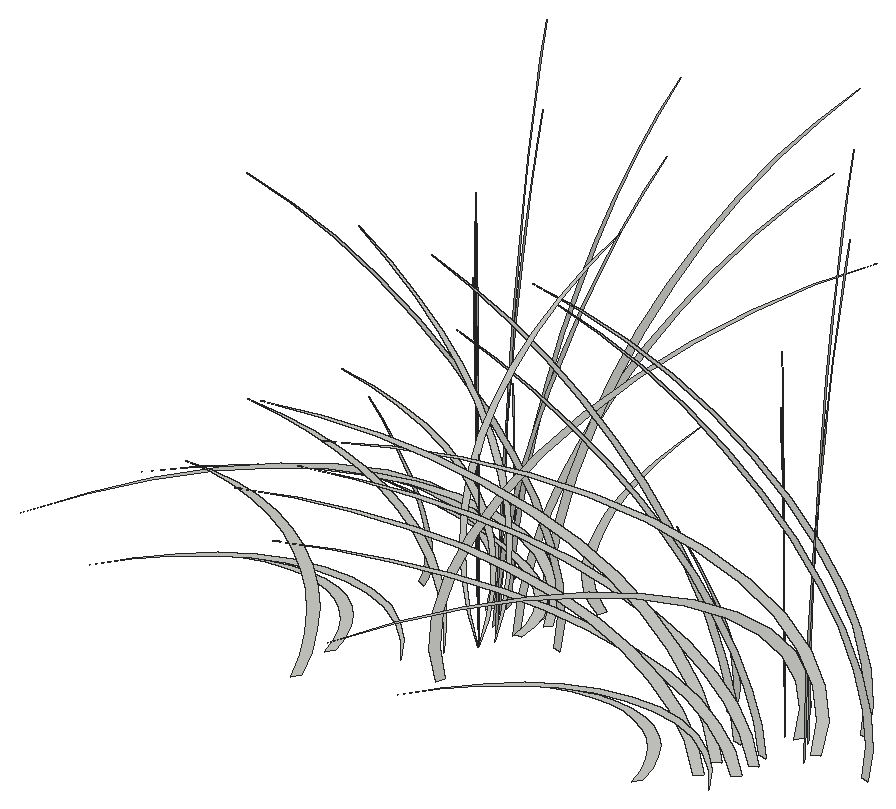
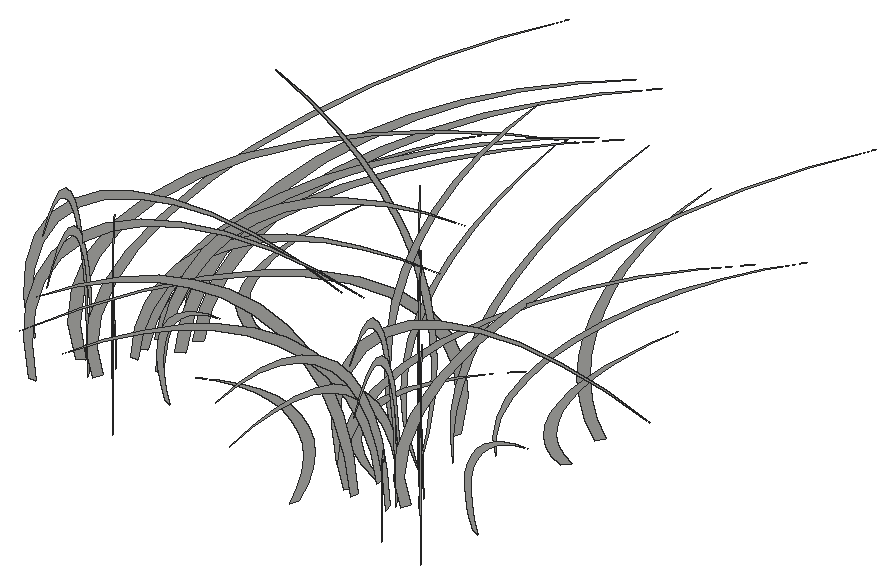
# SketchUp Ruby script. Lengths in inches.
U = 1.inch
M = Sketchup.active_model
def pt(a) = Geom::Point3d.new(a.map { |v| v * U })
def face(e, loops, mat)
  f = e.add_face(loops[0].map { |a| pt(a) })
  loops[1..].each { |l| e.add_face(l.map { |a| pt(a) }).erase! }
  f.material = f.back_material = mat if mat
  f
end
# faces: each face lists its corners as indices into pts; further lists are holes
def faces(e, pts, list, mat = nil) = list.each { |f| face(e, (f[0].is_a?(Array) ? f : [f]).map { |l| l.map { |i| pts[i] } }, mat) }
# xy, xz, yz: faces in a plane at the given z, y or x. An outline is a flat list of corners, or four numbers for a rectangle; further outlines are holes
def ring(l) = l.size == 4 ? [[l[0], l[1]], [l[2], l[1]], [l[2], l[3]], [l[0], l[3]]] : l.each_slice(2).to_a
def flat(e, list, mat, &to3) = list.each { |f| face(e, (f[0].is_a?(Array) ? f : [f]).map { |l| ring(l).map { |u, v| to3.(u, v) } }, mat) }
def xy(e, z, list, mat = nil) = flat(e, list, mat) { |x, y| [x, y, z] }
def xz(e, y, list, mat = nil) = flat(e, list, mat) { |x, z| [x, y, z] }
def yz(e, x, list, mat = nil) = flat(e, list, mat) { |y, z| [x, y, z] }
def lines(e, pts, list) = list.each { |a, b| e.add_line(pt(pts[a]), pt(pts[b])) }
# prism: a flat outline (further loops are holes) pulled along v
def prism(e, loops, v, mat = nil)
  f = face(e, loops, mat); d = Geom::Vector3d.new(v.map { |x| x * U })
  f.pushpull(f.normal.samedirection?(d) ? d.length : -d.length)
end
def box(e, o, s, mat = nil) = prism(e, [[o, [o[0] + s[0], o[1], o[2]], [o[0] + s[0], o[1] + s[1], o[2]], [o[0], o[1] + s[1], o[2]]]], [0, 0, s[2]], mat)
def at(x, y, z, deg = 0) = Geom::Transformation.translation(pt([x, y, z])) * Geom::Transformation.rotation(ORIGIN, Z_AXIS, deg.degrees)
def axes(o, x, y, z) = Geom::Transformation.new([*x, 0, *y, 0, *z, 0, *pt(o).to_a, 1])
def part(name) = M.definitions.add(name)
# library, detail: a bought-in or finely detailed component or shape, given as its bounding box
def library(name, o, s) = part(name).tap { |d| box(d.entities, o, s) }
def detail(e, o, s) = box(e.add_group.entities, o, s)
def put(e, d, t, mat = nil) = e.add_instance(d, t).tap { |i| i.material = mat if mat }
def group(e, t, mat = nil) = e.add_group.tap { |g| g.transformation = t; g.material = mat if mat }.entities
root = M.entities
g1 = group(root,at(461.7,262.6875,0))
p = [[-0.95,0.28,0],[-0.42,0.125,0],[0,0,2.01],[-0.17,0.05,4.04],[-0.93,0.27,6.02],[-2.27,0.66,7.92],
  [-4.14,1.21,9.68],[-6.5,1.9,11.26],[-9.3,2.72,12.62],[-12.46,3.64,13.73],[-15.91,4.65,14.5625],[-19.55,5.72,15.09],
  [-23.3125,6.82,15.31],[-27.08,7.92,15.2],[-23.38,6.84,15.22],[-19.72,5.77,14.94],[-16.17,4.73,14.37],[-12.83,3.75,13.51],
  [-9.77,2.86,12.39],[-7.0625,2.07,11.04],[-4.77,1.39,9.48],[-2.94,0.86,7.75],[-1.62,0.47,5.9],[-0.84,0.25,3.96],
  [-0.61,0.18,1.98]]
faces(g1,p,[[0,1,2,3,4,5,6,7,8,9,10,11,12,13,14,15,16,17,18,19,20,21,22,23,24]])
g2 = group(root,at(452.43,263.44,0))
p = [[-6.53,2.99,7.88],[-5.33,2.44,7.38],[-4.26,1.95,6.83],[-3.3,1.51,6.24],[-2.48,1.14,5.62],[-1.81,0.83,4.96],
  [-1.28,0.58,4.27],[-0.9,0.41,3.57],[-0.68,0.31,2.86],[-0.61,0.28,2.13],[-0.71,0.32,1.41],[-0.96,0.4375,0.7],
  [-1.37,0.625,0],[-0.84,0.38,0],[-0.39,0.18,0.71],[-0.11,0.05,1.43],[0,0,2.17],[-0.07,0.03,2.9],
  [-0.32,0.15,3.63],[-0.74,0.34,4.34],[-1.33,0.61,5.03],[-2.08,0.95,5.69],[-2.99,1.37,6.3125],[-4.04,1.85,6.89],
  [-5.22,2.39,7.41]]
faces(g2,p,[[0,1,2,3,4,5,6,7,8,9,10,11,12,13,14,15,16,17,18,19,20,21,22,23,24]])
g3 = group(root,at(455.19,263.66,0))
p = [[-10.66,12.98,9.9],[-9.23,11.23,9.83],[-7.82,9.52,9.59],[-6.46,7.86,9.18],[-5.18,6.3,8.61],[-3.99,4.86,7.88],
  [-2.93,3.57,7.02],[-2.02,2.46,6.03],[-1.27,1.54,4.95],[-0.6875,0.84,3.78],[-0.29,0.36,2.55],[-0.1,0.12,1.28],
  [-0.09,0.12,0],[0,0,1.3],[-0.125,0.15,2.61],[-0.47,0.57,3.875],[-1.02,1.24,5.09],[-1.77,2.15,6.21],
  [-2.69,3.28,7.22],[-3.78,4.6,8.1],[-5,6.09,8.82],[-6.33,7.71,9.37],[-7.74,9.43,9.74],[-9.2,11.19,9.92]]
faces(g3,p,[[0,1,2,3,4,5,6,7,8,9,10,11,12,13,14,15,16,17,18,19,20,21,22,23]])
g4 = group(root,at(456.45,263.9375,0))
p = [[-11.32,17.43,20.75],[-13.02,20.05,21.3],[-11.37,17.51,20.63],[-9.77,15.05,19.72],[-8.25,12.7,18.55],[-6.82,10.5,17.16],
  [-5.5,8.46,15.55],[-4.29,6.61,13.74],[-3.23,4.97,11.76],[-2.3125,3.56,9.62],[-1.55,2.39,7.35],[-0.96,1.47,4.97],
  [-0.54,0.83,2.51],[-0.29,0.45,0],[0,0,0],[-0.2,0.31,2.57],[-0.59,0.91,5.09],[-1.18,1.8125,7.53],
  [-1.94,2.99,9.85],[-2.88,4.43,12.03],[-3.98,6.12,14.04],[-5.22,8.04,15.86],[-6.59,10.15,17.46],[-8.08,12.44,18.82],
  [-9.66,14.88,19.92]]
faces(g4,p,[[0,1,2,3,4,5,6,7,8,9,10,11,12,13,14,15,16,17,18,19,20,21,22,23,24]])
g5 = group(root,at(452.33,267.16,0))
p = [[-4.56,5.55,16.02],[-3.72,4.53,15.01],[-2.97,3.62,13.89],[-2.31,2.81,12.69],[-1.73,2.11,11.42],[-1.26,1.54,10.08],
  [-0.89,1.09,8.6875],[-0.63,0.76,7.26],[-0.47,0.58,5.8],[-0.43,0.52,4.34],[-0.49,0.6,2.87],[-0.67,0.81,1.42],
  [-0.95,1.16,0],[-0.59,0.71,0],[-0.27,0.33,1.44],[-0.07,0.09,2.92],[0,0,4.41],[-0.05,0.0625,5.9],
  [-0.22,0.27,7.38],[-0.52,0.63,8.83],[-0.93,1.13,10.23],[-1.45,1.77,11.57],[-2.09,2.54,12.83],[-2.82,3.43,14.01],
  [-3.65,4.44,15.07]]
faces(g5,p,[[0,1,2,3,4,5,6,7,8,9,10,11,12,13,14,15,16,17,18,19,20,21,22,23,24]])
g6 = group(root,at(452.33,267.16,0))
p = [[-4.56,5.55,16.02],[-3.72,4.53,15.01],[-2.97,3.62,13.89],[-2.31,2.81,12.69],[-1.73,2.11,11.42],[-1.26,1.54,10.08],
  [-0.89,1.09,8.6875],[-0.63,0.76,7.26],[-0.47,0.58,5.8],[-0.43,0.52,4.34],[-0.49,0.6,2.87],[-0.67,0.81,1.42],
  [-0.95,1.16,0],[-0.59,0.71,0],[-0.27,0.33,1.44],[-0.07,0.09,2.92],[0,0,4.41],[-0.05,0.0625,5.9],
  [-0.22,0.27,7.38],[-0.52,0.63,8.83],[-0.93,1.13,10.23],[-1.45,1.77,11.57],[-2.09,2.54,12.83],[-2.82,3.43,14.01],
  [-3.65,4.44,15.07]]
faces(g6,p,[[0,1,2,3,4,5,6,7,8,9,10,11,12,13,14,15,16,17,18,19,20,21,22,23,24]])
g7 = group(root,at(456.02,264.74,0))
p = [[-0.37,-0.92,0],[-0.16,-0.41,0],[0,0,1.75],[-0.07,-0.17,3.51],[-0.36,-0.9,5.24],[-0.88,-2.19,6.89],
  [-1.61,-4,8.42],[-2.53,-6.28,9.8],[-3.61,-8.99,10.98],[-4.84,-12.04,11.95],[-6.18,-15.375,12.67],[-7.6,-18.9,13.13],
  [-9.06,-22.53,13.32],[-10.53,-26.18,13.23],[-9.09,-22.6,13.25],[-7.66,-19.06,13],[-6.29,-15.63,12.5],[-4.99,-12.41,11.75],
  [-3.8,-9.45,10.78],[-2.75,-6.83,9.6],[-1.85,-4.61,8.25],[-1.14,-2.84,6.75],[-0.63,-1.57,5.13],[-0.33,-0.8125,3.44],
  [-0.24,-0.59,1.72]]
faces(g7,p,[[0,1,2,3,4,5,6,7,8,9,10,11,12,13,14,15,16,17,18,19,20,21,22,23,24]])
g8 = group(root,at(452.77,256.56,0))
p = [[-3.94,-6,6.7],[-3.22,-4.9,6.27],[-2.57,-3.91,5.81],[-2,-3.04,5.31],[-1.5,-2.28,4.77],[-1.09,-1.66,4.21],
  [-0.77,-1.17,3.63],[-0.54,-0.83,3.03],[-0.41,-0.62,2.43],[-0.37,-0.5625,1.8125],[-0.43,-0.65,1.2],[-0.58,-0.88,0.59],
  [-0.83,-1.26,0],[-0.51,-0.77,0],[-0.23,-0.36,0.6],[-0.0625,-0.1,1.22],[0,0,1.84],[-0.04,-0.07,2.47],
  [-0.19,-0.29,3.09],[-0.45,-0.68,3.69],[-0.8,-1.22,4.28],[-1.26,-1.91,4.84],[-1.81,-2.75,5.37],[-2.44,-3.71,5.86],
  [-3.16,-4.8,6.3]]
faces(g8,p,[[0,1,2,3,4,5,6,7,8,9,10,11,12,13,14,15,16,17,18,19,20,21,22,23,24]])
g9 = group(root,at(455.54,257.25,0))
p = [[-9.23,-14.04,8.41],[-7.99,-12.15,8.36],[-6.77,-10.29,8.15],[-5.59,-8.5,7.8],[-4.48,-6.8125,7.32],[-3.46,-5.26,6.7],
  [-2.54,-3.86,5.97],[-1.75,-2.66,5.13],[-1.09,-1.67,4.2],[-0.59,-0.9,3.21],[-0.25,-0.39,2.16],[-0.08,-0.125,1.09],
  [-0.08,-0.125,0],[0,0,1.11],[-0.11,-0.16,2.21],[-0.4,-0.61,3.29],[-0.88,-1.34,4.32],[-1.53,-2.33,5.28],
  [-2.33,-3.55,6.14],[-3.27,-4.98,6.88],[-4.33,-6.59,7.5],[-5.48,-8.34,7.97],[-6.7,-10.19,8.28],[-7.96,-12.11,8.43]]
faces(g9,p,[[0,1,2,3,4,5,6,7,8,9,10,11,12,13,14,15,16,17,18,19,20,21,22,23]])
g10 = group(root,at(457.5,262.32,0))
p = [[-11.32,17.43,16.73],[-13.02,20.05,17.17],[-11.37,17.51,16.64],[-9.77,15.05,15.9],[-8.25,12.7,14.96],[-6.82,10.5,13.84],
  [-5.5,8.46,12.54],[-4.29,6.61,11.08],[-3.23,4.97,9.48],[-2.3125,3.56,7.76],[-1.55,2.39,5.92],[-0.96,1.47,4.01],
  [-0.54,0.83,2.02],[-0.29,0.45,0],[0,0,0],[-0.2,0.31,2.07],[-0.59,0.91,4.1],[-1.18,1.8125,6.07],
  [-1.94,2.99,7.94],[-2.88,4.43,9.7],[-3.98,6.12,11.33],[-5.22,8.04,12.79],[-6.59,10.15,14.08],[-8.08,12.44,15.17],
  [-9.66,14.88,16.0625]]
faces(g10,p,[[0,1,2,3,4,5,6,7,8,9,10,11,12,13,14,15,16,17,18,19,20,21,22,23,24]])
g11 = group(root,at(453.05,253.48,0))
p = [[-3.94,-6,13.62],[-3.22,-4.9,12.76],[-2.57,-3.91,11.81],[-2,-3.04,10.79],[-1.5,-2.28,9.7],[-1.09,-1.66,8.57],
  [-0.77,-1.17,7.38],[-0.54,-0.83,6.17],[-0.41,-0.62,4.93],[-0.37,-0.5625,3.6875],[-0.43,-0.65,2.44],[-0.58,-0.88,1.21],
  [-0.83,-1.26,0],[-0.51,-0.77,0],[-0.23,-0.36,1.22],[-0.0625,-0.1,2.48],[0,0,3.75],[-0.04,-0.07,5.02],
  [-0.19,-0.29,6.28],[-0.45,-0.68,7.51],[-0.8,-1.22,8.7],[-1.26,-1.91,9.84],[-1.81,-2.75,10.91],[-2.44,-3.71,11.9],
  [-3.16,-4.8,12.8125]]
faces(g11,p,[[0,1,2,3,4,5,6,7,8,9,10,11,12,13,14,15,16,17,18,19,20,21,22,23,24]])
g12 = group(root,at(459.52,264.9,0))
p = [[-0.5,-0.57,0],[-0.22,-0.25,0],[0,0,1.46],[-0.09,-0.1,2.93],[-0.49,-0.56,4.375],[-1.19,-1.35,5.75],
  [-2.17,-2.47,7.03],[-3.41,-3.89,8.18],[-4.88,-5.56,9.17],[-6.54,-7.45,9.98],[-8.36,-9.51,10.58],[-10.27,-11.69,10.97],
  [-12.24,-13.9375,11.125],[-14.23,-16.19,11.05],[-12.28,-13.98,11.0625],[-10.36,-11.79,10.86],[-8.5,-9.67,10.44],[-6.74,-7.67,9.82],
  [-5.13,-5.84,9.01],[-3.71,-4.22,8.02],[-2.51,-2.85,6.89],[-1.54,-1.76,5.64],[-0.85,-0.97,4.29],[-0.44,-0.5,2.88],
  [-0.32,-0.37,1.4375]]
faces(g12,p,[[0,1,2,3,4,5,6,7,8,9,10,11,12,13,14,15,16,17,18,19,20,21,22,23,24]])
g13 = group(root,at(459.52,264.9,0))
p = [[-0.5,-0.57,0],[-0.22,-0.25,0],[0,0,1.46],[-0.09,-0.1,2.93],[-0.49,-0.56,4.375],[-1.19,-1.35,5.75],
  [-2.17,-2.47,7.03],[-3.41,-3.89,8.18],[-4.88,-5.56,9.17],[-6.54,-7.45,9.98],[-8.36,-9.51,10.58],[-10.27,-11.69,10.97],
  [-12.24,-13.9375,11.125],[-14.23,-16.19,11.05],[-12.28,-13.98,11.0625],[-10.36,-11.79,10.86],[-8.5,-9.67,10.44],[-6.74,-7.67,9.82],
  [-5.13,-5.84,9.01],[-3.71,-4.22,8.02],[-2.51,-2.85,6.89],[-1.54,-1.76,5.64],[-0.85,-0.97,4.29],[-0.44,-0.5,2.88],
  [-0.32,-0.37,1.4375]]
faces(g13,p,[[0,1,2,3,4,5,6,7,8,9,10,11,12,13,14,15,16,17,18,19,20,21,22,23,24]])
g14 = group(root,at(456.41,264.57,0))
p = [[-6.07,19.87,18.05],[-6.99,22.87,18.53],[-6.1,19.96,17.95],[-5.25,17.16,17.15],[-4.43,14.49,16.14],[-3.66,11.97,14.93],
  [-2.95,9.65,13.53],[-2.31,7.54,11.96],[-1.73,5.67,10.23],[-1.24,4.06,8.37],[-0.83,2.72,6.39],[-0.51,1.68,4.32],
  [-0.29,0.94,2.18],[-0.16,0.52,0],[0,0,0],[-0.11,0.35,2.23],[-0.32,1.04,4.43],[-0.63,2.07,6.55],
  [-1.04,3.41,8.57],[-1.55,5.05,10.47],[-2.13,6.98,12.22],[-2.8,9.16,13.8],[-3.54,11.58,15.1875],[-4.34,14.1875,16.37],
  [-5.1875,16.96,17.33]]
faces(g14,p,[[0,1,2,3,4,5,6,7,8,9,10,11,12,13,14,15,16,17,18,19,20,21,22,23,24]])
g15 = group(root,at(455.35,266.52,0))
p = [[-4.56,5.55,7.88],[-3.72,4.53,7.38],[-2.97,3.62,6.83],[-2.31,2.81,6.24],[-1.73,2.11,5.62],[-1.26,1.54,4.96],
  [-0.89,1.09,4.27],[-0.63,0.76,3.57],[-0.47,0.58,2.86],[-0.43,0.52,2.13],[-0.49,0.6,1.41],[-0.67,0.81,0.7],
  [-0.95,1.16,0],[-0.59,0.71,0],[-0.27,0.33,0.71],[-0.07,0.09,1.43],[0,0,2.17],[-0.05,0.0625,2.9],
  [-0.22,0.27,3.63],[-0.52,0.63,4.34],[-0.93,1.13,5.03],[-1.45,1.77,5.69],[-2.09,2.54,6.3125],[-2.82,3.43,6.89],
  [-3.65,4.44,7.41]]
faces(g15,p,[[0,1,2,3,4,5,6,7,8,9,10,11,12,13,14,15,16,17,18,19,20,21,22,23,24]])
g16 = group(root,at(456.64,261.91,0))
p = [[-6.74,8.21,19.61],[-5.67,6.9,18.16],[-4.68,5.7,16.67],[-3.78,4.6,15.125],[-2.98,3.62,13.55],[-2.27,2.76,11.93],
  [-1.65,2.01,10.28],[-1.14,1.39,8.61],[-0.72,0.88,6.91],[-0.41,0.5,5.2],[-0.2,0.24,3.47],[-0.09,0.11,1.74],
  [-0.09,0.11,0],[0,0,1.74],[-0.03,0.04,3.49],[-0.1875,0.23,5.23],[-0.46,0.56,6.96],[-0.85,1.04,8.67],
  [-1.36,1.66,10.36],[-1.98,2.42,12.01],[-2.72,3.3125,13.63],[-3.57,4.35,15.21],[-4.52,5.51,16.73],[-5.58,6.8,18.2]]
faces(g16,p,[[0,1,2,3,4,5,6,7,8,9,10,11,12,13,14,15,16,17,18,19,20,21,22,23]])
g17 = group(root,at(456.64,261.91,0))
p = [[-6.74,8.21,19.61],[-5.67,6.9,18.16],[-4.68,5.7,16.67],[-3.78,4.6,15.125],[-2.98,3.62,13.55],[-2.27,2.76,11.93],
  [-1.65,2.01,10.28],[-1.14,1.39,8.61],[-0.72,0.88,6.91],[-0.41,0.5,5.2],[-0.2,0.24,3.47],[-0.09,0.11,1.74],
  [-0.09,0.11,0],[0,0,1.74],[-0.03,0.04,3.49],[-0.1875,0.23,5.23],[-0.46,0.56,6.96],[-0.85,1.04,8.67],
  [-1.36,1.66,10.36],[-1.98,2.42,12.01],[-2.72,3.3125,13.63],[-3.57,4.35,15.21],[-4.52,5.51,16.73],[-5.58,6.8,18.2]]
faces(g17,p,[[0,1,2,3,4,5,6,7,8,9,10,11,12,13,14,15,16,17,18,19,20,21,22,23]])
g18 = group(root,at(456.98,262.72,0))
p = [[-6.07,19.87,14.56],[-6.99,22.87,14.94],[-6.1,19.96,14.48],[-5.25,17.16,13.83],[-4.43,14.49,13.02],[-3.66,11.97,12.04],
  [-2.95,9.65,10.91],[-2.31,7.54,9.64],[-1.73,5.67,8.25],[-1.24,4.06,6.75],[-0.83,2.72,5.15],[-0.51,1.68,3.49],
  [-0.29,0.94,1.76],[-0.16,0.52,0],[0,0,0],[-0.11,0.35,1.8],[-0.32,1.04,3.57],[-0.63,2.07,5.28],
  [-1.04,3.41,6.91],[-1.55,5.05,8.44],[-2.13,6.98,9.85],[-2.8,9.16,11.13],[-3.54,11.58,12.25],[-4.34,14.1875,13.2],
  [-5.1875,16.96,13.97]]
faces(g18,p,[[0,1,2,3,4,5,6,7,8,9,10,11,12,13,14,15,16,17,18,19,20,21,22,23,24]])
g19 = group(root,at(456.78,259.15,0))
p = [[-5.83,-8.875,16.67],[-4.9,-7.46,15.44],[-4.05,-6.16,14.17],[-3.27,-4.98,12.86],[-2.58,-3.92,11.51],[-1.96,-2.98,10.14],
  [-1.43,-2.18,8.74],[-0.99,-1.5,7.31],[-0.63,-0.95,5.87],[-0.36,-0.54,4.42],[-0.17,-0.26,2.95],[-0.08,-0.12,1.48],
  [-0.08,-0.12,0],[0,0,1.48],[-0.03,-0.04,2.97],[-0.16,-0.24,4.45],[-0.4,-0.6,5.92],[-0.74,-1.12,7.37],
  [-1.18,-1.79,8.81],[-1.72,-2.61,10.21],[-2.36,-3.58,11.59],[-3.09,-4.7,12.93],[-3.92,-5.96,14.22],[-4.83,-7.35,15.47]]
faces(g19,p,[[0,1,2,3,4,5,6,7,8,9,10,11,12,13,14,15,16,17,18,19,20,21,22,23]])
g20 = group(root,at(458.89,261.88,0))
p = [[-0.89,-0.32,0],[-0.4,-0.14,1.97],[-0.1,-0.04,3.96],[0,0,5.95],[-0.1,-0.03,7.95],[-0.39,-0.14,9.9375],
  [-0.89,-0.3125,11.91],[-1.57,-0.56,13.85],[-2.45,-0.87,15.76],[-3.52,-1.25,17.63],[-4.77,-1.6875,19.44],[-6.19,-2.19,21.2],
  [-7.79,-2.76,22.89],[-6.29,-2.23,21.17],[-4.94,-1.75,19.4],[-3.76,-1.33,17.58],[-2.74,-0.97,15.71],[-1.89,-0.67,13.8],
  [-1.22,-0.43,11.86],[-0.72,-0.25,9.9],[-0.4,-0.14,7.93],[-0.25,-0.09,5.94],[-0.29,-0.1,3.95],[-0.5,-0.18,1.97]]
faces(g20,p,[[0,1,2,3,4,5,6,7,8,9,10,11,12,13,14,15,16,17,18,19,20,21,22,23]])
g21 = group(root,at(459.99,263.24,0))
p = [[-9.01,-2.98,7.88],[-7.3,-2.41,7.38],[-5.75,-1.9,6.83],[-4.38,-1.45,6.24],[-3.2,-1.06,5.62],[-2.23,-0.74,4.96],
  [-1.47,-0.49,4.27],[-0.92,-0.31,3.57],[-0.61,-0.2,2.86],[-0.51,-0.17,2.13],[-0.65,-0.21,1.41],[-1.01,-0.33,0.7],
  [-1.6,-0.53,0],[-1.21,-0.4,0],[-0.54,-0.18,0.69],[-0.12,-0.04,1.4],[0.06,0.02,2.13],[-0.02,-0.01,2.85],
  [-0.35,-0.11,3.58],[-0.92,-0.3,4.29],[-1.73,-0.57,4.98],[-2.78,-0.92,5.64],[-4.05,-1.34,6.27],[-5.52,-1.82,6.86],
  [-7.18,-2.375,7.4]]
faces(g21,p,[[0,1,2,3,4,5,6,7,8,9,10,11,12,13,14,15,16,17,18,19,20,21,22,23,24]])
g22 = group(root,at(458.33,259.85,0))
p = [[-0.6,0.73,0],[-0.27,0.33,1.77],[-0.07,0.08,3.57],[0,0,5.36],[-0.07,0.08,7.16],[-0.27,0.32,8.95],
  [-0.6,0.73,10.73],[-1.06,1.29,12.48],[-1.65,2.01,14.2],[-2.37,2.88,15.88],[-3.21,3.91,17.52],[-4.17,5.08,19.1],
  [-5.25,6.39,20.625],[-4.23,5.15,19.08],[-3.33,4.05,17.48],[-2.53,3.08,15.83],[-1.84,2.25,14.15],[-1.27,1.55,12.43],
  [-0.82,1,10.6875],[-0.48,0.59,8.92],[-0.27,0.32,7.14],[-0.17,0.21,5.35],[-0.19,0.24,3.5625],[-0.34,0.41,1.78]]
faces(g22,p,[[0,1,2,3,4,5,6,7,8,9,10,11,12,13,14,15,16,17,18,19,20,21,22,23]])
g23 = group(root,at(458.25,261.375,0))
p = [[-0.52,-0.79,0],[-0.23,-0.35,1.51],[-0.06,-0.09,3.03],[0,0,4.56],[-0.06,-0.09,6.09],[-0.23,-0.35,7.61],
  [-0.52,-0.79,9.12],[-0.92,-1.39,10.61],[-1.43,-2.17,12.07],[-2.05,-3.12,13.5],[-2.78,-4.23,14.89],[-3.61,-5.49,16.24],
  [-4.54,-6.91,17.53],[-3.66,-5.57,16.21],[-2.88,-4.38,14.86],[-2.1875,-3.33,13.46],[-1.6,-2.43,12.03],[-1.1,-1.68,10.57],
  [-0.71,-1.08,9.08],[-0.42,-0.64,7.58],[-0.23,-0.35,6.07],[-0.15,-0.22,4.55],[-0.17,-0.25,3.03],[-0.29,-0.44,1.51]]
faces(g23,p,[[0,1,2,3,4,5,6,7,8,9,10,11,12,13,14,15,16,17,18,19,20,21,22,23]])
g24 = group(root,at(458.35,262.61,0))
p = [[1.63,20.71,16.73],[1.875,23.84,17.17],[1.64,20.8125,16.64],[1.41,17.89,15.9],[1.1875,15.1,14.96],[0.98,12.48,13.84],
  [0.79,10.06,12.54],[0.62,7.86,11.08],[0.47,5.91,9.48],[0.33,4.23,7.76],[0.22,2.84,5.92],[0.14,1.75,4.01],
  [0.08,0.98,2.02],[0.04,0.54,0],[0,0,0],[0.03,0.36,2.07],[0.09,1.09,4.1],[0.17,2.15,6.07],
  [0.28,3.55,7.94],[0.41,5.27,9.7],[0.57,7.28,11.33],[0.75,9.55,12.79],[0.95,12.07,14.08],[1.16,14.79,15.17],
  [1.39,17.68,16.0625]]
faces(g24,p,[[0,1,2,3,4,5,6,7,8,9,10,11,12,13,14,15,16,17,18,19,20,21,22,23,24]])
g25 = group(root,at(458.5,264.53,0))
p = [[1.63,20.71,20.75],[1.875,23.84,21.3],[1.64,20.8125,20.63],[1.41,17.89,19.72],[1.1875,15.1,18.55],[0.98,12.48,17.16],
  [0.79,10.06,15.55],[0.62,7.86,13.74],[0.47,5.91,11.76],[0.33,4.23,9.62],[0.22,2.84,7.35],[0.14,1.75,4.97],
  [0.08,0.98,2.51],[0.04,0.54,0],[0,0,0],[0.03,0.36,2.57],[0.09,1.09,5.09],[0.17,2.15,7.53],
  [0.28,3.55,9.85],[0.41,5.27,12.03],[0.57,7.28,14.04],[0.75,9.55,15.86],[0.95,12.07,17.46],[1.16,14.79,18.82],
  [1.39,17.68,19.92]]
faces(g25,p,[[0,1,2,3,4,5,6,7,8,9,10,11,12,13,14,15,16,17,18,19,20,21,22,23,24]])
g26 = group(root,at(457.05,259.91,0))
p = [[0.67,0.67,0],[0.3,0.3,2.04],[0.08,0.08,4.1],[0,0,6.17],[0.07,0.07,8.23],[0.3,0.3,10.29],
  [0.66,0.66,12.33],[1.18,1.18,14.34],[1.84,1.84,16.32],[2.64,2.64,18.26],[3.58,3.58,20.14],[4.65,4.65,21.96],
  [5.84,5.84,23.71],[4.72,4.72,21.93],[3.71,3.71,20.09],[2.82,2.82,18.2],[2.05,2.05,16.26],[1.42,1.42,14.29],
  [0.91,0.91,12.29],[0.54,0.54,10.26],[0.3,0.3,8.21],[0.1875,0.1875,6.15],[0.22,0.22,4.09],[0.375,0.375,2.04]]
faces(g26,p,[[0,1,2,3,4,5,6,7,8,9,10,11,12,13,14,15,16,17,18,19,20,21,22,23]])
g27 = group(root,at(460.04,266.13,0))
p = [[2.34,6.79,9.0625],[1.91,5.55,8.49],[1.52,4.43,7.85],[1.18,3.44,7.18],[0.89,2.58,6.45],[0.65,1.88,5.7],
  [0.46,1.33,4.91],[0.32,0.93,4.1],[0.24,0.7,3.28],[0.22,0.64,2.45],[0.25,0.74,1.625],[0.34,1,0.8],
  [0.49,1.42,0],[0.3,0.875,0],[0.14,0.4,0.81],[0.04,0.11,1.65],[0,0,2.49],[0.03,0.07,3.34],
  [0.11,0.33,4.17],[0.27,0.77,4.99],[0.48,1.38,5.79],[0.75,2.17,6.54],[1.07,3.11,7.26],[1.45,4.2,7.92],
  [1.87,5.43,8.52]]
faces(g27,p,[[0,1,2,3,4,5,6,7,8,9,10,11,12,13,14,15,16,17,18,19,20,21,22,23,24]])
g28 = group(root,at(458.2,255.98,0))
p = [[0.26,0.96,0],[0.11,0.43,0],[0,0,2.01],[0.05,0.17,4.04],[0.25,0.9375,6.02],[0.62,2.28,7.92],
  [1.125,4.16,9.68],[1.76,6.54,11.26],[2.52,9.35,12.62],[3.38,12.53,13.73],[4.32,16,14.5625],[5.31,19.67,15.09],
  [6.33,23.45,15.31],[7.35,27.24,15.2],[6.35,23.52,15.22],[5.35,19.83,14.94],[4.39,16.27,14.37],[3.48,12.91,13.51],
  [2.65,9.83,12.39],[1.92,7.11,11.04],[1.29,4.8,9.48],[0.8,2.96,7.75],[0.44,1.63,5.9],[0.23,0.84,3.96],
  [0.17,0.62,1.98]]
faces(g28,p,[[0,1,2,3,4,5,6,7,8,9,10,11,12,13,14,15,16,17,18,19,20,21,22,23,24]])
g29 = group(root,at(474.53,260.99,0))
p = [[-20.46,3.64,18.05],[-23.54,4.19,18.53],[-20.55,3.66,17.95],[-17.67,3.15,17.15],[-14.91,2.66,16.14],[-12.33,2.2,14.93],
  [-9.93,1.77,13.53],[-7.76,1.38,11.96],[-5.84,1.04,10.23],[-4.18,0.74,8.37],[-2.8,0.5,6.39],[-1.73,0.31,4.32],
  [-0.97,0.17,2.18],[-0.53,0.09,0],[0,0,0],[-0.36,0.0625,2.23],[-1.07,0.19,4.43],[-2.125,0.38,6.55],
  [-3.51,0.625,8.57],[-5.2,0.93,10.47],[-7.1875,1.28,12.22],[-9.43,1.68,13.8],[-11.92,2.125,15.1875],[-14.61,2.6,16.37],
  [-17.46,3.11,17.33]]
faces(g29,p,[[0,1,2,3,4,5,6,7,8,9,10,11,12,13,14,15,16,17,18,19,20,21,22,23,24]])
g30 = group(root,at(474.92,258.89,0))
p = [[-18.45,-9.5625,18.05],[-21.23,-11,18.53],[-18.53,-9.61,17.95],[-15.93,-8.26,17.15],[-13.45,-6.97,16.14],[-11.12,-5.76,14.93],
  [-8.96,-4.64,13.53],[-7,-3.63,11.96],[-5.26,-2.73,10.23],[-3.77,-1.95,8.37],[-2.53,-1.3125,6.39],[-1.5625,-0.81,4.32],
  [-0.875,-0.45,2.18],[-0.48,-0.25,0],[0,0,0],[-0.32,-0.17,2.23],[-0.97,-0.5,4.43],[-1.92,-0.99,6.55],
  [-3.16,-1.64,8.57],[-4.69,-2.43,10.47],[-6.48,-3.36,12.22],[-8.51,-4.41,13.8],[-10.75,-5.57,15.1875],[-13.17,-6.83,16.37],
  [-15.75,-8.16,17.33]]
faces(g30,p,[[0,1,2,3,4,5,6,7,8,9,10,11,12,13,14,15,16,17,18,19,20,21,22,23,24]])
g31 = group(root,at(474.92,258.89,0))
p = [[-18.45,-9.5625,18.05],[-21.23,-11,18.53],[-18.53,-9.61,17.95],[-15.93,-8.26,17.15],[-13.45,-6.97,16.14],[-11.12,-5.76,14.93],
  [-8.96,-4.64,13.53],[-7,-3.63,11.96],[-5.26,-2.73,10.23],[-3.77,-1.95,8.37],[-2.53,-1.3125,6.39],[-1.5625,-0.81,4.32],
  [-0.875,-0.45,2.18],[-0.48,-0.25,0],[0,0,0],[-0.32,-0.17,2.23],[-0.97,-0.5,4.43],[-1.92,-0.99,6.55],
  [-3.16,-1.64,8.57],[-4.69,-2.43,10.47],[-6.48,-3.36,12.22],[-8.51,-4.41,13.8],[-10.75,-5.57,15.1875],[-13.17,-6.83,16.37],
  [-15.75,-8.16,17.33]]
faces(g31,p,[[0,1,2,3,4,5,6,7,8,9,10,11,12,13,14,15,16,17,18,19,20,21,22,23,24]])
g32 = group(root,at(476.43,260.65,0))
p = [[-20.46,3.64,14.56],[-23.54,4.19,14.94],[-20.55,3.66,14.48],[-17.67,3.15,13.83],[-14.91,2.66,13.02],[-12.33,2.2,12.04],
  [-9.93,1.77,10.91],[-7.76,1.38,9.64],[-5.84,1.04,8.25],[-4.18,0.74,6.75],[-2.8,0.5,5.15],[-1.73,0.31,3.49],
  [-0.97,0.17,1.76],[-0.53,0.09,0],[0,0,0],[-0.36,0.0625,1.8],[-1.07,0.19,3.57],[-2.125,0.38,5.28],
  [-3.51,0.625,6.91],[-5.2,0.93,8.44],[-7.1875,1.28,9.85],[-9.43,1.68,11.13],[-11.92,2.125,12.25],[-14.61,2.6,13.2],
  [-17.46,3.11,13.97]]
faces(g32,p,[[0,1,2,3,4,5,6,7,8,9,10,11,12,13,14,15,16,17,18,19,20,21,22,23,24]])
g33 = group(root,at(474.97,257.39,0))
p = [[-17.17,-11.7,15.34],[-19.76,-13.47,15.75],[-17.25,-11.76,15.26],[-14.83,-10.11,14.58],[-12.52,-8.53,13.72],[-10.35,-7.05,12.69],
  [-8.34,-5.68,11.5],[-6.52,-4.44,10.16],[-4.9,-3.34,8.7],[-3.51,-2.39,7.11],[-2.35,-1.6,5.43],[-1.45,-0.99,3.67],
  [-0.82,-0.56,1.86],[-0.45,-0.3,0],[0,0,0],[-0.3,-0.21,1.9],[-0.9,-0.61,3.76],[-1.78,-1.22,5.57],
  [-2.95,-2.01,7.28],[-4.37,-2.98,8.9],[-6.03,-4.11,10.39],[-7.92,-5.4,11.73],[-10,-6.82,12.91],[-12.26,-8.36,13.91],
  [-14.66,-9.99,14.73]]
faces(g33,p,[[0,1,2,3,4,5,6,7,8,9,10,11,12,13,14,15,16,17,18,19,20,21,22,23,24]])
g34 = group(root,at(476.64,259.78,0))
p = [[-18.45,-9.5625,14.56],[-21.23,-11,14.94],[-18.53,-9.61,14.48],[-15.93,-8.26,13.83],[-13.45,-6.97,13.02],[-11.12,-5.76,12.04],
  [-8.96,-4.64,10.91],[-7,-3.63,9.64],[-5.26,-2.73,8.25],[-3.77,-1.95,6.75],[-2.53,-1.3125,5.15],[-1.5625,-0.81,3.49],
  [-0.875,-0.45,1.76],[-0.48,-0.25,0],[0,0,0],[-0.32,-0.17,1.8],[-0.97,-0.5,3.57],[-1.92,-0.99,5.28],
  [-3.16,-1.64,6.91],[-4.69,-2.43,8.44],[-6.48,-3.36,9.85],[-8.51,-4.41,11.13],[-10.75,-5.57,12.25],[-13.17,-6.83,13.2],
  [-15.75,-8.16,13.97]]
faces(g34,p,[[0,1,2,3,4,5,6,7,8,9,10,11,12,13,14,15,16,17,18,19,20,21,22,23,24]])
g35 = group(root,at(476.64,259.78,0))
p = [[-18.45,-9.5625,14.56],[-21.23,-11,14.94],[-18.53,-9.61,14.48],[-15.93,-8.26,13.83],[-13.45,-6.97,13.02],[-11.12,-5.76,12.04],
  [-8.96,-4.64,10.91],[-7,-3.63,9.64],[-5.26,-2.73,8.25],[-3.77,-1.95,6.75],[-2.53,-1.3125,5.15],[-1.5625,-0.81,3.49],
  [-0.875,-0.45,1.76],[-0.48,-0.25,0],[0,0,0],[-0.32,-0.17,1.8],[-0.97,-0.5,3.57],[-1.92,-0.99,5.28],
  [-3.16,-1.64,6.91],[-4.69,-2.43,8.44],[-6.48,-3.36,9.85],[-8.51,-4.41,11.13],[-10.75,-5.57,12.25],[-13.17,-6.83,13.2],
  [-15.75,-8.16,13.97]]
faces(g35,p,[[0,1,2,3,4,5,6,7,8,9,10,11,12,13,14,15,16,17,18,19,20,21,22,23,24]])
g36 = group(root,at(479.5,265.5,0))
p = [[-0.91,0.16,0],[-0.4,0.07,0],[0,0,2.0625],[-0.16,0.03,4.13],[-0.89,0.16,6.16],[-2.17,0.39,8.1],
  [-3.95,0.7,9.91],[-6.21,1.11,11.52],[-8.88,1.58,12.92],[-11.91,2.12,14.05],[-15.2,2.71,14.9],[-18.68,3.33,15.45],
  [-22.27,3.97,15.67],[-25.88,4.61,15.5625],[-22.34,3.98,15.58],[-18.84,3.36,15.29],[-15.45,2.75,14.71],[-12.26,2.18,13.83],
  [-9.34,1.66,12.68],[-6.75,1.2,11.3],[-4.56,0.8125,9.7],[-2.81,0.5,7.9375],[-1.55,0.28,6.04],[-0.8,0.14,4.05],
  [-0.59,0.1,2.02]]
faces(g36,p,[[0,1,2,3,4,5,6,7,8,9,10,11,12,13,14,15,16,17,18,19,20,21,22,23,24]])
g37 = group(root,at(479.5,265.5,0))
p = [[-0.91,0.16,0],[-0.4,0.07,0],[0,0,2.0625],[-0.16,0.03,4.13],[-0.89,0.16,6.16],[-2.17,0.39,8.1],
  [-3.95,0.7,9.91],[-6.21,1.11,11.52],[-8.88,1.58,12.92],[-11.91,2.12,14.05],[-15.2,2.71,14.9],[-18.68,3.33,15.45],
  [-22.27,3.97,15.67],[-25.88,4.61,15.5625],[-22.34,3.98,15.58],[-18.84,3.36,15.29],[-15.45,2.75,14.71],[-12.26,2.18,13.83],
  [-9.34,1.66,12.68],[-6.75,1.2,11.3],[-4.56,0.8125,9.7],[-2.81,0.5,7.9375],[-1.55,0.28,6.04],[-0.8,0.14,4.05],
  [-0.59,0.1,2.02]]
faces(g37,p,[[0,1,2,3,4,5,6,7,8,9,10,11,12,13,14,15,16,17,18,19,20,21,22,23,24]])
g38 = group(root,at(476.5625,258.48,0))
p = [[-17.17,-11.7,12.375],[-19.76,-13.47,12.7],[-17.25,-11.76,12.31],[-14.83,-10.11,11.76],[-12.52,-8.53,11.07],[-10.35,-7.05,10.23],
  [-8.34,-5.68,9.27],[-6.52,-4.44,8.2],[-4.9,-3.34,7.01],[-3.51,-2.39,5.74],[-2.35,-1.6,4.38],[-1.45,-0.99,2.96],
  [-0.82,-0.56,1.5],[-0.45,-0.3,0],[0,0,0],[-0.3,-0.21,1.53],[-0.9,-0.61,3.03],[-1.78,-1.22,4.49],
  [-2.95,-2.01,5.875],[-4.37,-2.98,7.18],[-6.03,-4.11,8.375],[-7.92,-5.4,9.46],[-10,-6.82,10.41],[-12.26,-8.36,11.22],
  [-14.66,-9.99,11.88]]
faces(g38,p,[[0,1,2,3,4,5,6,7,8,9,10,11,12,13,14,15,16,17,18,19,20,21,22,23,24]])
g39 = group(root,at(478.76,262.8,0))
p = [[-0.82,-0.43,0],[-0.36,-0.1875,0],[0,0,2.0625],[-0.15,-0.08,4.13],[-0.8,-0.42,6.16],[-1.95,-1.01,8.1],
  [-3.57,-1.85,9.91],[-5.6,-2.9,11.52],[-8.01,-4.15,12.92],[-10.74,-5.57,14.05],[-13.71,-7.1,14.9],[-16.85,-8.73,15.45],
  [-20.09,-10.41,15.67],[-23.34,-12.1,15.5625],[-20.15,-10.44,15.58],[-16.99,-8.81,15.29],[-13.9375,-7.22,14.71],[-11.06,-5.73,13.83],
  [-8.42,-4.37,12.68],[-6.09,-3.16,11.3],[-4.11,-2.13,9.7],[-2.53,-1.3125,7.9375],[-1.4,-0.72,6.04],[-0.72,-0.375,4.05],
  [-0.53,-0.27,2.02]]
faces(g39,p,[[0,1,2,3,4,5,6,7,8,9,10,11,12,13,14,15,16,17,18,19,20,21,22,23,24]])
g40 = group(root,at(482.36,261.93,0))
p = [[-0.95,0.28,0],[-0.42,0.125,0],[0,0,2.01],[-0.17,0.05,4.04],[-0.93,0.27,6.02],[-2.27,0.66,7.92],
  [-4.14,1.21,9.68],[-6.5,1.9,11.26],[-9.3,2.72,12.62],[-12.46,3.64,13.73],[-15.91,4.65,14.5625],[-19.55,5.72,15.09],
  [-23.3125,6.82,15.31],[-27.08,7.92,15.2],[-23.38,6.84,15.22],[-19.72,5.77,14.94],[-16.17,4.73,14.37],[-12.83,3.75,13.51],
  [-9.77,2.86,12.39],[-7.0625,2.07,11.04],[-4.77,1.39,9.48],[-2.94,0.86,7.75],[-1.62,0.47,5.9],[-0.84,0.25,3.96],
  [-0.61,0.18,1.98]]
faces(g40,p,[[0,1,2,3,4,5,6,7,8,9,10,11,12,13,14,15,16,17,18,19,20,21,22,23,24]])
g41 = group(root,at(473.09,262.68,0))
p = [[-6.53,2.99,7.88],[-5.33,2.44,7.38],[-4.26,1.95,6.83],[-3.3,1.51,6.24],[-2.48,1.14,5.62],[-1.81,0.83,4.96],
  [-1.28,0.58,4.27],[-0.9,0.41,3.57],[-0.68,0.31,2.86],[-0.61,0.28,2.13],[-0.71,0.32,1.41],[-0.96,0.4375,0.7],
  [-1.37,0.625,0],[-0.84,0.38,0],[-0.39,0.18,0.71],[-0.11,0.05,1.43],[0,0,2.17],[-0.07,0.03,2.9],
  [-0.32,0.15,3.63],[-0.74,0.34,4.34],[-1.33,0.61,5.03],[-2.08,0.95,5.69],[-2.99,1.37,6.3125],[-4.04,1.85,6.89],
  [-5.22,2.39,7.41]]
faces(g41,p,[[0,1,2,3,4,5,6,7,8,9,10,11,12,13,14,15,16,17,18,19,20,21,22,23,24]])
g42 = group(root,at(475.85,262.91,0))
p = [[-10.66,12.98,9.9],[-9.23,11.23,9.83],[-7.82,9.52,9.59],[-6.46,7.86,9.18],[-5.18,6.3,8.61],[-3.99,4.86,7.88],
  [-2.93,3.57,7.02],[-2.02,2.46,6.03],[-1.27,1.54,4.95],[-0.6875,0.84,3.78],[-0.29,0.36,2.55],[-0.1,0.12,1.28],
  [-0.09,0.12,0],[0,0,1.3],[-0.125,0.15,2.61],[-0.47,0.57,3.875],[-1.02,1.24,5.09],[-1.77,2.15,6.21],
  [-2.69,3.28,7.22],[-3.78,4.6,8.1],[-5,6.09,8.82],[-6.33,7.71,9.37],[-7.74,9.43,9.74],[-9.2,11.19,9.92]]
faces(g42,p,[[0,1,2,3,4,5,6,7,8,9,10,11,12,13,14,15,16,17,18,19,20,21,22,23]])
g43 = group(root,at(477.11,263.18,0))
p = [[-11.32,17.43,20.75],[-13.02,20.05,21.3],[-11.37,17.51,20.63],[-9.77,15.05,19.72],[-8.25,12.7,18.55],[-6.82,10.5,17.16],
  [-5.5,8.46,15.55],[-4.29,6.61,13.74],[-3.23,4.97,11.76],[-2.3125,3.56,9.62],[-1.55,2.39,7.35],[-0.96,1.47,4.97],
  [-0.54,0.83,2.51],[-0.29,0.45,0],[0,0,0],[-0.2,0.31,2.57],[-0.59,0.91,5.09],[-1.18,1.8125,7.53],
  [-1.94,2.99,9.85],[-2.88,4.43,12.03],[-3.98,6.12,14.04],[-5.22,8.04,15.86],[-6.59,10.15,17.46],[-8.08,12.44,18.82],
  [-9.66,14.88,19.92]]
faces(g43,p,[[0,1,2,3,4,5,6,7,8,9,10,11,12,13,14,15,16,17,18,19,20,21,22,23,24]])
g44 = group(root,at(472.99,266.4,0))
p = [[-4.56,5.55,16.02],[-3.72,4.53,15.01],[-2.97,3.62,13.89],[-2.31,2.81,12.69],[-1.73,2.11,11.42],[-1.26,1.54,10.08],
  [-0.89,1.09,8.6875],[-0.63,0.76,7.26],[-0.47,0.58,5.8],[-0.43,0.52,4.34],[-0.49,0.6,2.87],[-0.67,0.81,1.42],
  [-0.95,1.16,0],[-0.59,0.71,0],[-0.27,0.33,1.44],[-0.07,0.09,2.92],[0,0,4.41],[-0.05,0.0625,5.9],
  [-0.22,0.27,7.38],[-0.52,0.63,8.83],[-0.93,1.13,10.23],[-1.45,1.77,11.57],[-2.09,2.54,12.83],[-2.82,3.43,14.01],
  [-3.65,4.44,15.07]]
faces(g44,p,[[0,1,2,3,4,5,6,7,8,9,10,11,12,13,14,15,16,17,18,19,20,21,22,23,24]])
g45 = group(root,at(472.99,266.4,0))
p = [[-4.56,5.55,16.02],[-3.72,4.53,15.01],[-2.97,3.62,13.89],[-2.31,2.81,12.69],[-1.73,2.11,11.42],[-1.26,1.54,10.08],
  [-0.89,1.09,8.6875],[-0.63,0.76,7.26],[-0.47,0.58,5.8],[-0.43,0.52,4.34],[-0.49,0.6,2.87],[-0.67,0.81,1.42],
  [-0.95,1.16,0],[-0.59,0.71,0],[-0.27,0.33,1.44],[-0.07,0.09,2.92],[0,0,4.41],[-0.05,0.0625,5.9],
  [-0.22,0.27,7.38],[-0.52,0.63,8.83],[-0.93,1.13,10.23],[-1.45,1.77,11.57],[-2.09,2.54,12.83],[-2.82,3.43,14.01],
  [-3.65,4.44,15.07]]
faces(g45,p,[[0,1,2,3,4,5,6,7,8,9,10,11,12,13,14,15,16,17,18,19,20,21,22,23,24]])
g46 = group(root,at(476.68,263.99,0))
p = [[-0.37,-0.92,0],[-0.16,-0.41,0],[0,0,1.75],[-0.07,-0.17,3.51],[-0.36,-0.9,5.24],[-0.88,-2.19,6.89],
  [-1.61,-4,8.42],[-2.53,-6.28,9.8],[-3.61,-8.99,10.98],[-4.84,-12.04,11.95],[-6.18,-15.375,12.67],[-7.6,-18.9,13.13],
  [-9.06,-22.53,13.32],[-10.53,-26.18,13.23],[-9.09,-22.6,13.25],[-7.66,-19.06,13],[-6.29,-15.63,12.5],[-4.99,-12.41,11.75],
  [-3.8,-9.45,10.78],[-2.75,-6.83,9.6],[-1.85,-4.61,8.25],[-1.14,-2.84,6.75],[-0.63,-1.57,5.13],[-0.33,-0.8125,3.44],
  [-0.24,-0.59,1.72]]
faces(g46,p,[[0,1,2,3,4,5,6,7,8,9,10,11,12,13,14,15,16,17,18,19,20,21,22,23,24]])
g47 = group(root,at(473.42,255.8,0))
p = [[-3.94,-6,6.7],[-3.22,-4.9,6.27],[-2.57,-3.91,5.81],[-2,-3.04,5.31],[-1.5,-2.28,4.77],[-1.09,-1.66,4.21],
  [-0.77,-1.17,3.63],[-0.54,-0.83,3.03],[-0.41,-0.62,2.43],[-0.37,-0.5625,1.8125],[-0.43,-0.65,1.2],[-0.58,-0.88,0.59],
  [-0.83,-1.26,0],[-0.51,-0.77,0],[-0.23,-0.36,0.6],[-0.0625,-0.1,1.22],[0,0,1.84],[-0.04,-0.07,2.47],
  [-0.19,-0.29,3.09],[-0.45,-0.68,3.69],[-0.8,-1.22,4.28],[-1.26,-1.91,4.84],[-1.81,-2.75,5.37],[-2.44,-3.71,5.86],
  [-3.16,-4.8,6.3]]
faces(g47,p,[[0,1,2,3,4,5,6,7,8,9,10,11,12,13,14,15,16,17,18,19,20,21,22,23,24]])
g48 = group(root,at(476.19,256.5,0))
p = [[-9.23,-14.04,8.41],[-7.99,-12.15,8.36],[-6.77,-10.29,8.15],[-5.59,-8.5,7.8],[-4.48,-6.8125,7.32],[-3.46,-5.26,6.7],
  [-2.54,-3.86,5.97],[-1.75,-2.66,5.13],[-1.09,-1.67,4.2],[-0.59,-0.9,3.21],[-0.25,-0.39,2.16],[-0.08,-0.125,1.09],
  [-0.08,-0.125,0],[0,0,1.11],[-0.11,-0.16,2.21],[-0.4,-0.61,3.29],[-0.88,-1.34,4.32],[-1.53,-2.33,5.28],
  [-2.33,-3.55,6.14],[-3.27,-4.98,6.88],[-4.33,-6.59,7.5],[-5.48,-8.34,7.97],[-6.7,-10.19,8.28],[-7.96,-12.11,8.43]]
faces(g48,p,[[0,1,2,3,4,5,6,7,8,9,10,11,12,13,14,15,16,17,18,19,20,21,22,23]])
g49 = group(root,at(478.16,261.5625,0))
p = [[-11.32,17.43,16.73],[-13.02,20.05,17.17],[-11.37,17.51,16.64],[-9.77,15.05,15.9],[-8.25,12.7,14.96],[-6.82,10.5,13.84],
  [-5.5,8.46,12.54],[-4.29,6.61,11.08],[-3.23,4.97,9.48],[-2.3125,3.56,7.76],[-1.55,2.39,5.92],[-0.96,1.47,4.01],
  [-0.54,0.83,2.02],[-0.29,0.45,0],[0,0,0],[-0.2,0.31,2.07],[-0.59,0.91,4.1],[-1.18,1.8125,6.07],
  [-1.94,2.99,7.94],[-2.88,4.43,9.7],[-3.98,6.12,11.33],[-5.22,8.04,12.79],[-6.59,10.15,14.08],[-8.08,12.44,15.17],
  [-9.66,14.88,16.0625]]
faces(g49,p,[[0,1,2,3,4,5,6,7,8,9,10,11,12,13,14,15,16,17,18,19,20,21,22,23,24]])
